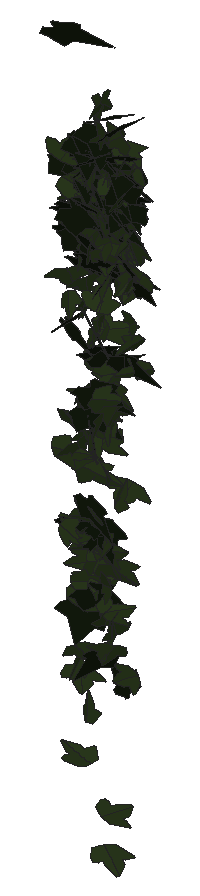
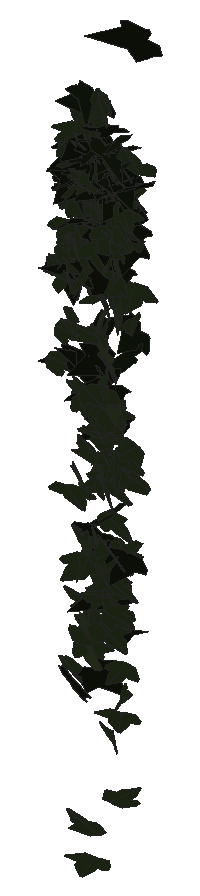
# SketchUp Ruby script. Lengths in millimetres.
U = 1.mm
M = Sketchup.active_model
def pt(a) = Geom::Point3d.new(a.map { |v| v * U })
def face(e, loops, mat)
  f = e.add_face(loops[0].map { |a| pt(a) })
  loops[1..].each { |l| e.add_face(l.map { |a| pt(a) }).erase! }
  f.material = f.back_material = mat if mat
  f
end
# faces: each face lists its corners as indices into pts; further lists are holes
def faces(e, pts, list, mat = nil) = list.each { |f| face(e, (f[0].is_a?(Array) ? f : [f]).map { |l| l.map { |i| pts[i] } }, mat) }
# xy, xz, yz: faces in a plane at the given z, y or x. An outline is a flat list of corners, or four numbers for a rectangle; further outlines are holes
def ring(l) = l.size == 4 ? [[l[0], l[1]], [l[2], l[1]], [l[2], l[3]], [l[0], l[3]]] : l.each_slice(2).to_a
def flat(e, list, mat, &to3) = list.each { |f| face(e, (f[0].is_a?(Array) ? f : [f]).map { |l| ring(l).map { |u, v| to3.(u, v) } }, mat) }
def xy(e, z, list, mat = nil) = flat(e, list, mat) { |x, y| [x, y, z] }
def xz(e, y, list, mat = nil) = flat(e, list, mat) { |x, z| [x, y, z] }
def yz(e, x, list, mat = nil) = flat(e, list, mat) { |y, z| [x, y, z] }
def lines(e, pts, list) = list.each { |a, b| e.add_line(pt(pts[a]), pt(pts[b])) }
# prism: a flat outline (further loops are holes) pulled along v
def prism(e, loops, v, mat = nil)
  f = face(e, loops, mat); d = Geom::Vector3d.new(v.map { |x| x * U })
  f.pushpull(f.normal.samedirection?(d) ? d.length : -d.length)
end
def box(e, o, s, mat = nil) = prism(e, [[o, [o[0] + s[0], o[1], o[2]], [o[0] + s[0], o[1] + s[1], o[2]], [o[0], o[1] + s[1], o[2]]]], [0, 0, s[2]], mat)
def at(x, y, z, deg = 0) = Geom::Transformation.translation(pt([x, y, z])) * Geom::Transformation.rotation(ORIGIN, Z_AXIS, deg.degrees)
def axes(o, x, y, z) = Geom::Transformation.new([*x, 0, *y, 0, *z, 0, *pt(o).to_a, 1])
def part(name) = M.definitions.add(name)
# library, detail: a bought-in or finely detailed component or shape, given as its bounding box
def library(name, o, s) = part(name).tap { |d| box(d.entities, o, s) }
def detail(e, o, s) = box(e.add_group.entities, o, s)
def put(e, d, t, mat = nil) = e.add_instance(d, t).tap { |i| i.material = mat if mat }
def group(e, t, mat = nil) = e.add_group.tap { |g| g.transformation = t; g.material = mat if mat }.entities
root = M.entities
M.materials.add("efeu1").color = [18, 25, 13]
M.materials.add("efeu2").color = [43, 57, 29]
c1 = part("ivyleaf_10")
p = [[0,12.8,-0.8],[-1.5,51.3,-10.9],[-4.9,51,-11.6],[-13.6,26.5,-7.3],[-13.2,15.9,-4.6],[-21.1,19.3,-7.2],
  [-29.5,16.3,-8.3],[-29.2,8.3,-6.2],[-19.7,-9.8,0.5],[-7.6,-13,4],[1,-12.2,5.8],[-0.4,51.1,-11.1],
  [-1.5,51.1,-10.9],[1,-12.4,5.9],[16.9,-12.4,3.5],[35.1,9.1,-5.1],[35,12.9,-6.1],[20.5,16.4,-4.9],
  [15.8,15,-3.8],[15.3,27.6,-7.1],[12.8,31.3,-7.8]]
faces(c1.entities,p,[[0,1,2,3,4,5,6,7,8,9,10],[11,12,0,13,14,15,16,17,18,19,20]],"efeu2")
c2 = part("ivyleaf_9")
p = [[39.1,54.8,31.7],[34.5,51.8,30.2],[-5.3,25.2,17.3],[-17.9,28.3,20.9],[-21.6,21.7,17],[-20.2,4.3,5.3],
  [-22.9,-0.3,2.5],[-17.1,-4,-0.6],[-2,-2.1,-1.2],[-0.7,-15.4,-10.1],[16.6,-22.3,-16.7],[21.1,-15.1,-12.5],
  [32.7,-10.7,-11],[46.1,-1.8,-6.6],[30.8,11.2,3.8]]
faces(c2.entities,p,[[0,1,2,3,4,5,6,7,8,9,10,11,12,13,14]],"efeu1")
put(root,c1,axes([2123.1,995.3,1030.1],[0.1906,0.68433,-0.17615],[-0.10749,-0.16959,-0.69095],[-1.34057,0.11089,0.03036]))
put(root,c1,axes([2125.7,988.9,1083.8],[-0.99593,-0.55975,-0.22734],[0.29957,0.16407,-0.76625],[1.11012,-0.54644,0.00281]))
put(root,c2,axes([2112.8,1000.5,1285.4],[0.02321,-0.74967,-0.23177],[0.08312,0.23208,-0.7484],[1.49109,-0.00127,0.04533]))
put(root,c1,axes([2135.8,1019.4,138.7],[0.62325,0.48649,0.41572],[-0.42495,-0.35077,0.58638],[1.14134,-0.39626,-0.00869]))
put(root,c1,axes([2116.7,1004.2,796.9],[-1.06583,0.27968,-0.34624],[0.60096,-0.14253,-0.62586],[-0.597,-0.6428,-0.01187]))
put(root,c1,axes([2133.1,1008.9,1242.5],[-0.27065,-0.75335,0.02688],[-0.01437,-0.02593,-0.76665],[1.43461,-0.14238,-0.00261]))
put(root,c1,axes([2133.3,1007.4,1229],[-0.52244,-0.70599,-0.01567],[0.01958,0.01282,-0.75747],[1.34384,-0.27465,0.00494]))
put(root,c1,axes([2102.9,999.1,731.2],[0.44156,-0.23226,-0.7183],[1.25411,-0.30437,0.31126],[-0.70107,-0.69076,0.10437]))
put(root,c2,axes([2126.7,1007.6,595.2],[1.22717,0.3981,-0.16174],[-0.27617,-0.07279,-0.75766],[-0.76976,0.66077,0.01398]))
put(root,c1,axes([2136.1,1008.7,1200.2],[-0.22378,-0.7354,0.18371],[-0.00371,-0.18561,-0.74427],[1.44263,-0.11455,0.02659]))
put(root,c2,axes([2113.8,1005.4,969.3],[0.92362,-0.62679,-0.07712],[-0.08881,0.0614,-0.79271],[1.19862,0.48754,0.00069]))
put(root,c1,axes([2125.4,1022,301.9],[1.17824,0.36942,0.04018],[0.0672,0.01923,-0.72092],[-0.70403,0.62009,-0.00157]))
put(root,c2,axes([2132.2,967.3,993.6],[0.46018,0.56096,0.59216],[0.42819,0.54781,-0.61081],[-1.49218,0.33019,0.00734]))
put(root,c1,axes([2142.9,1026.1,485.3],[-0.24172,-0.47422,0.54553],[-0.25536,-0.5288,-0.49091],[1.35179,-0.18469,0.00481]))
put(root,c1,axes([2121.2,985,1307.7],[1.44549,0.16265,-0.27372],[0.51115,0.05298,0.77672],[0.32546,-0.80558,-0.00418]))
put(root,c1,axes([2130.5,977.6,595.4],[-0.00655,0.62956,0.46716],[-0.00573,0.46715,-0.62957],[-1.49201,-0.00456,0.00037]))
put(root,c1,axes([2134.2,1010.4,326.8],[0.10382,0.30482,-0.67747],[-0.15658,-0.67264,-0.30927],[-1.40516,0.09747,-0.01559]))
put(root,c1,axes([2120.4,1016.4,708],[0.46974,-0.40499,-0.55279],[0.74794,-0.39768,0.46682],[-1.06843,-0.45645,0.08375]))
put(root,c1,axes([2141.8,994.7,756.5],[-0.48662,-0.77369,-0.37196],[0.19418,0.35797,-0.81472],[1.62223,-0.27493,-0.01405]))
put(root,c1,axes([2138.2,1015.5,847.5],[-0.26935,-0.35235,-0.59672],[-0.07607,-0.60387,0.36605],[-1.31668,0.10697,0.10092]))
put(root,c2,axes([2113.2,976.6,1550.7],[0.32292,0.23859,-0.77992],[0.84205,0.64229,0.29274],[1.30399,-0.47384,0.0041]))
put(root,c1,axes([2133.9,1002.4,588.8],[1.26574,0.16037,-0.13782],[0.25425,0.03394,0.68412],[0.31197,-0.67834,0.00164]))
put(root,c2,axes([2142.6,979.7,1166.2],[1.2367,0.10918,-0.4395],[-0.81863,-0.09161,-0.65872],[-0.26956,0.7791,-0.01587]))
put(root,c1,axes([2147.2,1006.1,1221.2],[-0.39847,-0.74045,0.0741],[-0.00265,-0.07659,-0.76923],[1.41625,-0.20847,0.01941]))
put(root,c2,axes([2157.8,999.7,1299.3],[0.47799,0.63308,-0.36755],[-0.67575,-0.23447,-0.64646],[-1.21837,0.37841,0.21435]))
put(root,c1,axes([2141.7,1033,569.8],[-0.05482,-0.12579,0.72322],[0.29785,-0.70819,-0.11695],[1.36497,0.14948,0.05457]))
put(root,c2,axes([2159.1,1006.5,1157.3],[-0.04924,0.08797,-0.81043],[-1.29872,0.44124,0.06968],[0.84874,0.68027,0.05961]))
put(root,c1,axes([2143,1015.2,1107.8],[-1.21258,0.36168,-0.0914],[0.13738,-0.05795,-0.73248],[-0.69658,-0.64103,0.01465]))
put(root,c2,axes([2118.9,984.6,1205.7],[1.17553,0.0895,0.47053],[0.86138,0.14223,-0.62117],[-0.29832,0.76333,0.06057]))
put(root,c2,axes([2162.2,992.1,1298.4],[-0.68201,0.68144,0.00431],[-0.00369,0.00385,-0.76992],[-1.29694,-0.35835,-0.00007]))
put(root,c1,axes([2166,1016.1,446.2],[-1.00082,-0.28656,0.45055],[-0.75452,-0.21406,-0.59887],[0.68074,-0.65856,-0.00139]))
put(root,c1,axes([2155.7,1021.7,837.1],[-0.36986,-0.36266,-0.60894],[-0.56519,-0.53165,0.4114],[-1.22477,0.35485,-0.00596]))
put(root,c2,axes([2145.3,993.3,1262.7],[0.74221,0.68815,0.26433],[0.24238,0.23165,-0.79097],[-1.38189,0.41023,0.00323]))
put(root,c2,axes([2148,991.1,1266.2],[-0.42561,0.72543,-0.3368],[-0.37212,0.28952,0.75342],[1.476,0.28217,0.09283]))
put(root,c1,axes([2152.7,1022.4,956.7],[0.42982,-0.64894,-0.08842],[-0.07411,0.08006,-0.68703],[1.24426,0.22894,-0.01038]))
put(root,c1,axes([2167.9,1006.7,536],[1.01125,-0.02957,-0.57194],[-1.08021,0.07698,-0.53127],[0.14553,0.77686,0.03087]))
put(root,c1,axes([2152,1015,773.9],[-0.55001,-0.67888,-0.2729],[0.19736,0.25245,-0.73782],[1.37847,-0.30702,-0.00325]))
put(root,c1,axes([2127.2,994.5,1184.1],[0.96208,-0.07101,0.60035],[1.14358,-0.02705,-0.50914],[0.12653,0.78437,0.0368]))
put(root,c1,axes([2164.3,1013.3,851.3],[-1.03656,-0.5294,0.27577],[-0.34253,-0.2103,-0.75917],[1.0832,-0.57311,0.02383]))
put(root,c1,axes([2147.3,989.4,369.2],[-0.72212,-0.41519,-0.37968],[0.49988,0.27427,-0.5624],[0.94693,-0.4614,0.00735]))
put(root,c1,axes([2156.6,1013.2,1192.5],[-1.15405,-0.43398,0.13134],[0.06766,-0.26416,-0.70869],[0.8603,-0.56139,0.23193]))
put(root,c2,axes([2177.1,998.4,590],[-0.88251,0.24143,-0.6951],[-1.21878,0.27227,0.52177],[0.68978,0.78996,0.0326]))
put(root,c2,axes([2150.6,1002.2,435],[-0.65061,-0.74582,0.11068],[-0.08528,-0.10121,-0.82043],[1.43245,-0.34477,0.00143]))
put(root,c1,axes([2157.8,1004.9,234.4],[0.95533,-0.45893,0.37581],[-0.52998,0.25238,0.68013],[-0.99679,-0.57402,-0.00143]))
put(root,c1,axes([2150.6,1007.2,1266.6],[-1.36192,-0.17808,-0.21029],[0.40464,0.01545,-0.73659],[0.33363,-0.74569,0.03496]))
put(root,c1,axes([2157.8,998.6,1173.6],[0.95469,-0.56592,-0.14151],[-0.11647,0.13455,-0.75503],[1.10409,0.50353,0.04271]))
put(root,c1,axes([2175.1,1006.7,574.7],[-0.55584,-0.33727,0.57779],[-0.73016,-0.43207,-0.44612],[1.04314,-0.48214,-0.00439]))
put(root,c1,axes([2163.7,1028.7,589.6],[-0.03045,0.00559,-0.7466],[-0.55334,-0.68787,0.00108],[-1.30881,0.29069,0.01691]))
put(root,c1,axes([2150.5,1000.7,1136.1],[0.27502,-0.54934,0.56919],[0.50438,-0.51155,-0.56099],[1.41851,0.2884,0.08912]))
put(root,c1,axes([2161.7,988.1,1045.2],[0.11245,-0.70184,-0.30774],[-0.03305,0.30735,-0.70428],[1.45814,0.06109,0.00777]))
put(root,c1,axes([2179.7,984.4,635.4],[-0.77726,0.02461,0.55664],[-1.059,0.01796,-0.40903],[-0.05528,-0.69016,0.00921]))
put(root,c2,axes([2150.1,1004.3,1279.9],[-0.3023,-0.75624,0.07728],[0.00329,-0.07931,-0.77254],[1.44677,-0.15784,0.0179]))
put(root,c2,axes([2151.9,1009.2,1305.1],[-0.35871,-0.55904,0.48848],[0.02664,-0.50656,-0.57433],[1.41265,-0.1324,0.13487]))
put(root,c1,axes([2148.3,988.7,1244.1],[-1.05643,0.30851,-0.44186],[0.6171,-0.31547,-0.62759],[-0.81921,-0.63548,0.09704]))
put(root,c1,axes([2164.8,983.9,1293],[1.01221,-0.50481,-0.2839],[-0.26448,0.26295,-0.72789],[1.07006,0.54251,0.08864]))
put(root,c2,axes([2175.6,997.9,1336.1],[-0.1106,0.75019,0.17904],[-0.21673,0.16924,-0.74607],[-1.45178,-0.08242,0.09774]))
put(root,c1,axes([2163,990.3,1034.1],[0.30569,-0.689,-0.23034],[0.01283,0.2373,-0.70514],[1.38258,0.15014,0.05747]))
put(root,c1,axes([2141.8,975.3,1266.6],[0.67684,0.39365,0.6463],[0.6837,0.54069,-0.52701],[-1.26761,0.50182,0.06084]))
put(root,c1,axes([2164.2,988.7,1082.4],[-0.54356,-0.66197,-0.21211],[0.14198,0.1988,-0.72089],[1.31532,-0.29502,-0.00984]))
put(root,c2,axes([2147.3,1005.5,1267],[0.48446,-0.68257,-0.23231],[0.0207,0.24997,-0.72254],[1.37209,0.23723,0.09293]))
put(root,c2,axes([2145.1,1005.3,1168.3],[0.49786,-0.68256,0.21834],[0.18302,-0.19689,-0.73074],[1.35156,0.27809,0.01853]))
put(root,c1,axes([2147.6,1032.1,914.7],[0.26893,-0.3027,0.65661],[0.96544,-0.43522,-0.30981],[0.98053,0.51155,0.12495]))
put(root,c1,axes([2166.1,1020.1,969.5],[0.49961,-0.6428,0.0458],[0.00844,-0.04765,-0.6942],[1.22645,0.26218,-0.01388]))
put(root,c1,axes([2169.2,1014.8,718.8],[0.54966,-0.68795,-0.15673],[-0.13164,0.14093,-0.74606],[1.3364,0.29684,-0.00903]))
put(root,c1,axes([2162.1,1004,1246.7],[0.99154,0.5584,-0.11091],[-0.16275,-0.07188,-0.76358],[-1.07121,0.52779,0.01335]))
put(root,c2,axes([2158.4,994.6,1333],[-0.33593,-0.75548,0.0174],[-0.00848,-0.01683,-0.77582],[1.43818,-0.17656,-0.00051]))
put(root,c1,axes([2172.8,987.7,1287.6],[0.72146,-0.62975,-0.27747],[-0.28767,0.23285,-0.73499],[1.27773,0.408,-0.00881]))
put(root,c1,axes([2187.9,1004.8,1153],[-0.5211,-0.07845,0.70308],[-0.92598,-0.52641,-0.24821],[0.97742,-0.54053,0.13969]))
put(root,c2,axes([2140.2,986.9,1218.1],[1.39496,-0.16802,0.24714],[0.45701,-0.05855,-0.75196],[0.33857,0.77128,-0.00324]))
put(root,c2,axes([2152,987.6,1166.4],[-0.07833,-0.51639,-0.61805],[0.27497,0.60408,-0.51434],[1.50793,-0.13698,0.06168]))
put(root,c1,axes([2169.5,999.3,1291.4],[-0.74225,-0.67294,-0.075],[0.16784,0.03533,-0.77559],[1.27768,-0.39557,0.05832]))
put(root,c1,axes([2176.8,1000.4,1243.2],[-1.14097,-0.44929,0.13192],[-0.19486,-0.08335,-0.74915],[0.86962,-0.60816,0.00522]))
put(root,c1,axes([2176.6,1019.9,1154.6],[-1.1965,-0.35651,0.14177],[-0.18423,-0.11595,-0.72085],[0.70657,-0.63395,0.05212]))
put(root,c1,axes([2156.4,1008.8,1308.5],[0.48105,-0.34799,0.63465],[0.71639,-0.51097,-0.43009],[1.17658,0.4534,0.0024]))
put(root,c1,axes([2169.5,1006.3,1270.5],[0.75682,-0.64727,-0.14511],[0.02721,0.17751,-0.75262],[1.26217,0.38429,0.10323]))
put(root,c1,axes([2183.6,1010.9,787.2],[1.0368,-0.07923,0.49181],[-0.92923,0.05969,0.55044],[-0.18813,-0.7315,-0.00835]))
put(root,c1,axes([2157.1,984.8,462.7],[1.25407,0.02388,-0.25657],[0.48791,0.01044,0.65936],[0.04956,-0.70704,0.00107]))
put(root,c2,axes([2154.3,1012.9,787.8],[0.02629,0.00313,-0.8044],[1.3086,-0.41761,0.01018],[-0.79459,-0.68765,-0.00985]))
put(root,c2,axes([2151.6,971.5,1220],[0.56113,-0.24248,-0.87086],[-0.02541,0.91474,-0.25922],[1.72029,0.0926,0.28023]))
put(root,c1,axes([2147.5,1012.8,816.4],[0.21865,-0.02257,0.68917],[1.06707,0.40976,-0.08004],[-0.76393,0.56591,0.08545]))
put(root,c1,axes([2183.9,988.4,1180.5],[-0.95323,-0.48174,0.2918],[-0.38061,-0.21293,-0.6948],[1.00207,-0.53913,0.01368]))
put(root,c2,axes([2159.7,1007.2,1259.6],[0.04829,-0.77043,-0.00224],[0.0002,0.00225,-0.77085],[1.46629,0.02537,0.00018]))
put(root,c1,axes([2158,979,503.9],[-0.09041,-0.0901,0.69977],[0.55632,0.63582,0.10171],[-1.22213,0.29609,-0.00547]))
put(root,c2,axes([2153.6,993.2,1348.2],[0.69333,-0.67624,-0.17594],[0.03274,0.20703,-0.76013],[1.32945,0.34757,0.11047]))
put(root,c1,axes([2164.2,1001.1,537.2],[-0.03287,-0.28581,-0.75932],[0.64334,0.6879,-0.26662],[1.40372,-0.32196,0.10441]))
put(root,c1,axes([2192.6,1003.3,714.8],[-0.39342,0.40739,-0.74788],[-0.74515,0.63798,0.45575],[1.4394,0.44162,0.03152]))
put(root,c1,axes([2171.8,1019,1161.8],[-1.28943,0.21779,0.21168],[0.35295,-0.11315,0.70997],[0.45776,0.70073,0.04885]))
put(root,c1,axes([2174.1,984.7,1151],[0.41329,-0.55667,-0.48039],[0.12294,0.51341,-0.56573],[1.39401,0.11976,0.19232]))
put(root,c1,axes([2170.1,1004.1,769.4],[0.096,0.73022,-0.15348],[-0.03878,-0.15243,-0.73189],[-1.41959,0.05355,0.00962]))
put(root,c1,axes([2191,994.7,1289.3],[0.73216,-0.29258,-0.59439],[-0.7721,0.43936,-0.47883],[0.99681,0.55521,0.06569]))
put(root,c1,axes([2181.4,1003.6,1157.1],[0.66119,-0.52139,-0.44504],[-0.19088,0.4549,-0.61123],[1.29059,0.3344,0.13759]))
put(root,c1,axes([2177.9,1004.1,1266.5],[0.49628,-0.72266,0.08953],[0.04653,-0.08636,-0.76825],[1.38511,0.26183,-0.00627]))
put(root,c1,axes([2173.1,994.7,1264.8],[-0.46184,0.69755,-0.19782],[0.05112,-0.19981,-0.73753],[-1.37898,-0.24103,0.03891]))
put(root,c1,axes([2178.7,983.8,1228.1],[-1.18814,0.42429,0.02489],[-0.04017,0.01322,-0.75482],[-0.8079,-0.62464,0.00093]))
put(root,c2,axes([2185.6,1000.6,1179.9],[0.94848,0.36695,-0.44053],[-0.83376,-0.13283,-0.60623],[-0.70393,0.65176,0.12447]))
put(root,c1,axes([2183.1,1007,1222.1],[-0.92806,-0.57572,0.15636],[0.03729,-0.2173,-0.73897],[1.13479,-0.46369,0.15216]))
put(root,c2,axes([2187.1,1010.8,362.1],[-0.17551,0.37815,-0.77973],[0.32176,-0.76122,-0.38917],[-1.61761,-0.19245,0.00719]))
put(root,c2,axes([2162.3,999.3,1275.4],[1.46887,0.05925,-0.00001],[-0.01481,0.10124,-0.76737],[-0.11179,0.76512,0.10154]))
put(root,c2,axes([2156.2,1007.1,1267.3],[0.97918,-0.57132,0.06293],[0.1617,-0.00793,-0.76667],[1.0819,0.51827,0.05764]))
put(root,c2,axes([2167.2,992.9,830.1],[0.0486,-0.42179,-0.76247],[-0.05173,0.76204,-0.42246],[1.65756,0.03615,0.00917]))
put(root,c2,axes([2185.3,986.3,1330.6],[0.75333,0.6132,-0.26896],[-0.31625,-0.21271,-0.7295],[-1.23451,0.42869,0.02275]))
put(root,c1,axes([2158.6,1001.8,589.5],[0.89619,0.11639,0.50683],[0.9124,0.16773,-0.48393],[-0.38344,0.67117,0.03305]))
put(root,c1,axes([2184.7,1008.9,990.1],[0.79388,-0.58263,-0.14501],[-0.16636,0.11576,-0.71655],[1.13052,0.42618,-0.00361]))
put(root,c2,axes([2156,986.3,1118.6],[1.48777,0.09078,0.29446],[0.55767,0.02943,-0.78696],[-0.18145,0.83482,-0.00428]))
put(root,c1,axes([2175.5,999.6,915.4],[1.33026,-0.30376,-0.00274],[0.0157,0.01211,0.76198],[-0.57792,-0.69886,0.01439]))
put(root,c1,axes([2185.7,997.7,1057.3],[0.64577,-0.66324,-0.11644],[-0.08367,0.10828,-0.74493],[1.27885,0.342,0.01006]))
put(root,c1,axes([2184.6,997.6,1014.8],[0.28272,-0.25111,-0.68556],[0.0687,0.70127,-0.24904],[1.38782,0.01644,0.15199]))
put(root,c2,axes([2183.4,971.1,1323.4],[0.53165,0.64425,0.33928],[0.23426,0.31637,-0.70211],[-1.36582,0.30504,0.01164]))
put(root,c2,axes([2166.4,992.6,651.7],[0.55686,-0.81264,-0.10232],[-0.071,0.09532,-0.8637],[1.55721,0.29495,-0.00279]))
put(root,c2,axes([2168.1,998.6,939.1],[0.96516,0.41395,0.46497],[0.70093,0.28402,-0.65454],[-0.95523,0.62666,-0.01049]))
put(root,c1,axes([2187.3,1029.1,888.7],[-0.44785,-0.55966,0.43975],[0.08175,-0.47348,-0.57961],[1.35216,-0.15674,0.18069]))
put(root,c1,axes([2186.7,997,1421.5],[0.70796,-0.66538,-0.21572],[-0.0477,0.23149,-0.75724],[1.33038,0.36238,0.08764]))
put(root,c1,axes([2175.3,1002.8,985.1],[0.11279,-0.18184,0.72332],[0.68897,-0.62738,-0.18738],[1.24104,0.36482,0.03829]))
put(root,c1,axes([2169.9,995.4,715.2],[-0.7575,-0.32731,-0.64646],[1.05864,0.33466,-0.51191],[0.88379,-0.68141,0.0591]))
put(root,c1,axes([2178.3,1007.7,583.9],[0.69578,-0.67525,-0.10081],[0.10554,-0.08461,0.76781],[-1.29508,-0.36967,0.00841]))
put(root,c1,axes([2188.6,998.3,1424.9],[-0.2161,-0.54971,-0.65849],[0.2113,0.64923,-0.56112],[1.6188,-0.15813,-0.01466]))
put(root,c1,axes([2181.8,1005.5,1252],[-1.10225,-0.4464,-0.25896],[0.6301,-0.02278,-0.70116],[0.75344,-0.63401,0.20752]))
put(root,c1,axes([2186.6,998.5,872.7],[-1.01391,-0.54992,-0.3576],[0.44192,0.27276,-0.76536],[1.16759,-0.58077,-0.02085]))
put(root,c1,axes([2193.3,1008.2,1245.4],[0.51263,-0.70136,-0.16635],[0.00118,0.17781,-0.74867],[1.37185,0.26193,0.0628]))
put(root,c1,axes([2196.1,1004.6,1280],[-0.68969,-0.6775,-0.10906],[0.09125,0.09803,-0.76832],[1.30283,-0.36552,-0.00392]))
put(root,c2,axes([2205.4,982.4,970.4],[0.0937,-0.60373,0.60557],[-0.12543,0.60209,0.60562],[-1.62259,-0.08141,-0.01185]))
put(root,c2,axes([2176.9,982.1,490.8],[0.0779,-0.11735,-0.80752],[0.17858,0.80385,-0.11206],[1.54272,-0.08713,0.05375]))
put(root,c1,axes([2208.2,992.6,1245.3],[-1.22569,0.18696,0.35491],[-0.68889,0.0185,-0.66657],[-0.32907,-0.7351,0.07349]))
put(root,c1,axes([2197.5,981.9,1390.3],[-0.94538,0.63448,0.0429],[-0.26187,-0.05409,-0.79328],[-1.18163,-0.49564,0.14148]))
put(root,c2,axes([2182.8,1003.4,613.1],[-0.96925,-0.22396,-0.63282],[1.11981,0.23345,-0.55613],[0.61501,-0.77802,0.01529]))
put(root,c1,axes([2185.5,992.9,492.9],[0.30836,0.2122,-0.76491],[0.62743,0.69219,0.26186],[1.37432,-0.36362,0.05208]))
put(root,c1,axes([2194.5,992.7,825.4],[0.255,-0.61287,0.3068],[0.19214,-0.29155,-0.62649],[1.29017,0.16455,0.03266]))
put(root,c2,axes([2193.4,998.2,1365.5],[-0.71121,-0.68913,-0.10923],[0.12241,0.08936,-0.78381],[1.32227,-0.37893,0.01381]))
put(root,c1,axes([2181.5,1018.5,761.6],[1.20984,-0.18503,-0.31988],[0.58245,-0.09313,0.66206],[-0.39418,-0.70551,-0.00351]))
put(root,c2,axes([2197.6,981.8,1076.3],[0.22269,0.22287,0.77167],[0.49419,0.72745,-0.24947],[-1.44659,0.28282,0.03357]))
put(root,c2,axes([2215.9,997.6,1214.4],[-0.56237,0.69132,0.10974],[-0.13024,0.09002,-0.75133],[-1.32581,-0.30208,0.02725]))
put(root,c1,axes([2203,1012.9,1141.1],[-1.04802,-0.49841,-0.0058],[0.00758,0.00425,-0.74272],[0.9486,-0.55068,-0.00048]))
put(root,c1,axes([2210.9,980.2,1173.2],[0.77695,-0.5559,-0.49614],[-0.57296,0.39444,-0.68965],[1.29718,0.50718,-0.00745]))
put(root,c1,axes([2188.2,1007.3,371.7],[0.35561,-0.71932,-0.25458],[0.27149,-0.22455,0.73917],[-1.42661,-0.22204,0.07721]))
put(root,c1,axes([2195.9,985.9,1045.1],[0.72784,0.66246,-0.36227],[0.29112,0.3297,0.76436],[1.40721,-0.41085,0.02925]))
put(root,c1,axes([2196.6,1007.3,1087.2],[0.02764,-0.60516,0.47972],[0.38609,-0.45996,-0.58638],[1.4181,0.13702,0.1503]))
put(root,c2,axes([2183.5,981.3,881.2],[0.08152,-0.2263,-0.77949],[0.31925,0.76619,-0.21322],[1.51144,-0.14963,0.08708]))
put(root,c1,axes([2190.6,999.3,1140.7],[1.37923,-0.04449,0.22869],[0.43373,-0.01976,-0.72603],[0.09205,0.75966,-0.0055]))
put(root,c1,axes([2201.6,1011.5,1220.9],[1.01797,-0.54169,-0.03414],[0.11055,0.10479,-0.75255],[1.02706,0.52562,0.11484]))
put(root,c1,axes([2202.4,1007,1299.1],[-1.07284,0.51328,-0.09591],[0.10259,-0.08318,-0.76197],[-0.98848,-0.56572,0.02501]))
put(root,c1,axes([2217.7,976.6,516.9],[0.463,-0.34808,-0.70701],[-0.51609,0.65777,-0.41714],[1.40823,0.3555,0.07958]))
put(root,c1,axes([2202.3,994.9,1309.3],[0.83177,-0.62924,0.18954],[0.20763,-0.155,-0.76612],[1.23336,0.45045,0.00115]))
put(root,c1,axes([2203.7,996.8,435.1],[-0.54556,-0.63728,-0.08889],[-0.02211,-0.09217,0.69826],[-1.22441,0.28561,0.027]))
put(root,c1,axes([2215.7,995.2,388.4],[-0.87986,-0.54099,0.17519],[-0.20398,-0.13885,-0.71156],[1.06285,-0.47449,0.00847]))
put(root,c1,axes([2195,1009.2,815.5],[0.86133,-0.45606,0.49666],[0.66542,-0.35274,-0.6425],[1.0973,0.57189,-0.00023]))
put(root,c1,axes([2213,997.7,1371.8],[-0.56541,-0.72355,-0.03236],[0.00584,0.03372,-0.7821],[1.37843,-0.29693,-0.00996]))
put(root,c2,axes([2176.9,1014.9,1105.1],[0.40855,0.06139,-0.8254],[1.07966,0.61001,0.19291],[1.14705,-0.59604,0.11241]))
put(root,c2,axes([2212.5,979.6,1409.4],[0.68089,0.63808,0.28206],[-0.07228,0.33433,-0.70815],[-1.32578,0.30948,0.18346]))
put(root,c1,axes([2207.5,998.9,1294],[-1.11273,0.51066,-0.08668],[0.13231,-0.05216,-0.77625],[-0.97686,-0.58874,-0.0064]))
put(root,c1,axes([2211.4,977.5,1215.5],[-0.24553,0.63164,0.40942],[-0.2557,0.38939,-0.64309],[-1.40958,-0.18066,0.04534]))
put(root,c2,axes([2191.8,998.8,919],[0.03699,-0.0347,0.76344],[1.375,0.24983,-0.00704],[-0.47422,0.72167,0.03915]))
put(root,c1,axes([2186,1011.9,985.5],[0.70331,-0.09053,-0.64841],[1.23932,0.12791,0.35326],[0.129,-0.73528,0.14129]))
put(root,c1,axes([2213,1010.9,411.7],[-0.39562,-0.64513,-0.35991],[-0.23494,-0.33829,0.67768],[-1.38618,0.24146,-0.01214]))
put(root,c1,axes([2219.6,997.7,847.1],[-0.73337,-0.60102,0.0939],[-0.0927,-0.08031,-0.71394],[1.15402,-0.3884,0.00232]))
put(root,c1,axes([2207.1,1010.1,430.6],[0.06475,-0.40387,-0.6787],[0.09063,-0.67704,0.40527],[-1.50036,-0.05832,-0.00481]))
put(root,c1,axes([2212.1,1018,1080.3],[-0.10512,0.71756,-0.02859],[-0.11244,-0.03311,-0.71706],[-1.3621,-0.05264,0.0614]))
put(root,c1,axes([2219,1000.9,548.5],[-0.24853,0.40394,0.56917],[-0.43256,0.52288,-0.42323],[-1.25593,-0.26002,0.03313]))
put(root,c1,axes([2211.5,1003,589.4],[0.13763,-0.35282,0.70235],[0.32744,-0.6811,-0.35986],[1.4596,0.18606,0.01451]))
put(root,c1,axes([2222.2,1007.7,1217.4],[-0.81626,-0.59636,0.21067],[-0.11533,-0.21463,-0.73091],[1.19819,-0.42692,0.07317]))
put(root,c1,axes([2218.5,1001.2,1254.8],[-0.06262,-0.6402,0.41441],[0.05549,-0.41555,-0.63964],[1.45036,-0.01174,0.04237]))
put(root,c1,axes([2203.1,997.6,-6.8],[1.08284,0.46628,0.22921],[0.33399,0.14748,-0.73561],[-0.93074,0.5954,0.0027]))
put(root,c2,axes([2197.6,997.5,1247.8],[0.5633,-0.69904,-0.00213],[0.07231,0.0184,-0.75794],[1.32845,0.29541,0.04216]))
put(root,c1,axes([2198.8,999.1,1255.5],[1.065,0.2124,-0.49753],[0.83585,0.2396,0.59624],[0.60117,-0.70941,0.05241]))
put(root,c1,axes([2195.9,1009.4,57.2],[0.98497,-0.03304,-0.47466],[0.90417,-0.00288,0.51819],[-0.05005,-0.70223,0.02021]))
put(root,c1,axes([2203.6,972.4,874.5],[-0.2548,-0.21487,-0.80094],[0.89747,0.64764,-0.25257],[1.29824,-0.48988,0.0174]))
put(root,c1,axes([2237.5,987.1,1378.1],[-0.91719,0.36232,0.49663],[-1.03667,0.04088,-0.55839],[-0.5424,-0.69081,0.22743]))
put(root,c2,axes([2216.4,1002.6,1280],[-0.88101,-0.60795,-0.10425],[0.14022,0.07492,-0.76401],[1.16553,-0.46855,0.01311]))
put(root,c2,axes([2199.2,1010.1,1199.8],[0.33384,-0.56337,-0.47937],[0.28181,0.50944,-0.54452],[1.37933,0.03227,0.22727]))
put(root,c2,axes([2202,1003.9,1323.9],[0.98661,-0.54014,-0.2023],[-0.17277,0.19221,-0.7458],[1.08404,0.52222,0.06526]))
put(root,c1,axes([2207.1,984.1,1153.5],[-0.7548,-0.30421,-0.61536],[0.96118,0.35203,-0.49952],[0.88485,-0.6419,0.01769]))
put(root,c1,axes([2196.8,997.1,571.8],[0.61027,-0.23828,-0.71476],[1.04555,-0.45766,0.39903],[-0.98131,-0.6358,-0.01935]))
put(root,c1,axes([2223.7,1015.6,1172.8],[-0.81024,-0.60612,-0.08955],[0.2228,0.02657,-0.73637],[1.14461,-0.43423,0.07995]))
put(root,c2,axes([2243.2,1005.4,315.9],[-0.1205,0.2723,0.7111],[-0.46066,0.66935,-0.27786],[-1.37403,-0.24829,0.0308]))
put(root,c1,axes([2238.6,1006.3,1153.1],[-0.13127,0.39523,0.63222],[-0.89794,0.4685,-0.34435],[-1.09877,-0.43008,0.20588]))
put(root,c1,axes([2228.2,1024.4,690.9],[1.39379,0.08478,-0.17386],[-0.33076,-0.01055,-0.73718],[-0.16165,0.75262,0.00925]))
put(root,c1,axes([2218.9,997.5,545.2],[-1.08504,-0.40213,-0.4742],[0.72376,0.28346,-0.69759],[0.93616,-0.68523,-0.01029]))
put(root,c1,axes([2208.9,1012.9,871.9],[-0.25907,0.09116,-0.71728],[0.83749,-0.5687,-0.15579],[-1.09192,-0.45782,0.0507]))
put(root,c2,axes([2218,982.8,1330.9],[0.96072,0.51406,0.27066],[0.39472,0.17547,-0.72008],[-1.03282,0.54524,-0.02344]))
put(root,c1,axes([2219.9,993.7,1284],[0.97747,0.65355,0.1581],[0.20053,0.11827,-0.83115],[-1.26391,0.5242,-0.0096]))
put(root,c2,axes([2204.3,1016.5,934],[0.0382,0.03924,-0.75868],[1.17951,0.43809,0.03906],[0.8362,-0.61974,-0.02043]))
put(root,c1,axes([2238.4,994.5,1215.8],[-1.05949,-0.4853,0.09085],[-0.12241,-0.06447,-0.7385],[0.93166,-0.56036,0.00629]))
put(root,c1,axes([2239.4,1016.1,1011.9],[0.62266,-0.42733,-0.45695],[-0.3614,0.42351,-0.53201],[1.13453,0.36943,0.08132]))
put(root,c1,axes([2234.2,1023.7,1086],[0.63892,-0.63345,-0.05716],[-0.01546,0.06036,-0.71661],[1.21039,0.33515,0.02102]))
put(root,c2,axes([2226.4,972.1,1389],[-0.17704,0.65707,-0.46318],[-0.19001,0.45322,0.66299],[1.51817,0.13335,0.02897]))
put(root,c1,axes([2240,1021.8,1137.5],[-0.58406,-0.6016,0.29864],[-0.05664,-0.31583,-0.66682],[1.27702,-0.28916,0.10701]))
put(root,c1,axes([2212.6,987.6,461.7],[0.80722,-0.03663,-0.54328],[1.03631,0.02951,0.42311],[0.00147,-0.6886,0.04703]))
put(root,c2,axes([2225.1,996.8,1259.2],[1.19842,0.41873,0.08048],[0.15228,0.02495,-0.75584],[-0.79711,0.63432,-0.0234]))
put(root,c1,axes([2233.4,1014.1,1158.6],[0.11605,0.73613,0.11685],[-0.09636,0.12106,-0.73623],[-1.41526,0.05212,0.05971]))
put(root,c1,axes([2236.7,996.8,1335.2],[0.54408,-0.73114,0.05065],[0.09157,-0.03552,-0.7844],[1.39184,0.28815,0.03181]))
put(root,c2,axes([2239.8,1006.4,1245.1],[-1.0532,-0.53924,-0.0067],[0.04411,-0.01419,-0.77222],[1.02542,-0.55324,0.02634]))
put(root,c2,axes([2231.8,992.8,1145.2],[1.17271,-0.18002,-0.4099],[-0.74846,0.11558,-0.64194],[0.40716,0.73098,0.00055]))
put(root,c1,axes([2253.8,1021.2,1102.6],[-1.15812,0.24593,0.34474],[-0.7746,-0.17298,-0.59501],[-0.22258,-0.67765,0.277]))
put(root,c1,axes([2234.4,1017.9,1168.4],[0.11225,-0.24793,0.70378],[0.31017,-0.68465,-0.25484],[1.38582,0.17332,0.00004]))
put(root,c2,axes([2251.5,977.5,1274.1],[-1.37674,0.34776,-0.12421],[-0.22102,0.04509,0.80258],[0.66714,0.73258,0.00956]))
put(root,c1,axes([2234.4,1011.4,1244.7],[-0.21852,0.73255,0.17535],[-0.03033,0.17498,-0.74141],[-1.43326,-0.11539,-0.01105]))
put(root,c2,axes([2246.7,1008.9,1096],[1.00106,0.1335,-0.60109],[-1.12729,-0.10625,-0.54191],[-0.32013,0.79163,0.02864]))
put(root,c1,axes([2242.8,1011.5,1099.7],[0.44882,0.47254,-0.49065],[-0.50177,-0.41545,-0.52682],[-1.19542,0.35179,0.03691]))
put(root,c1,axes([2242.3,987.9,1266.6],[0.08707,-0.7902,-0.24837],[0.02632,0.24944,-0.79106],[1.57622,0.03949,0.02693]))
put(root,c1,axes([2242.2,1028,1079],[-0.46877,-0.41245,0.52778],[0.09756,-0.57229,-0.42331],[1.27108,-0.10818,0.22714]))
put(root,c1,axes([2226.7,1019.5,1105.4],[-1.11561,0.09175,-0.43939],[0.7998,-0.14177,-0.59024],[-0.30019,-0.71872,0.06034]))
put(root,c2,axes([2222.4,998,1305.3],[1.42477,-0.18729,-0.03452],[-0.06304,0.00981,-0.77169],[0.35692,0.74935,0.00147]))
put(root,c1,axes([2252.7,999.4,346.4],[0.88119,-0.39093,-0.41607],[-0.62977,0.25279,-0.60574],[0.88544,0.56885,-0.01676]))
put(root,c1,axes([2242.2,1012.2,1095.5],[0.24509,-0.69831,-0.12199],[0.12311,0.13505,-0.70476],[1.34352,0.11501,0.08683]))
put(root,c1,axes([2255.9,1030,923.4],[-0.21147,-0.26039,0.66905],[-0.53847,-0.60634,-0.28297],[1.2558,-0.30384,-0.00867]))
put(root,c2,axes([2240.8,999.7,1322.6],[-0.77722,-0.67211,-0.04345],[0.03294,0.04032,-0.78643],[1.28141,-0.4087,-0.00614]))
put(root,c1,axes([2236.9,985.8,680.3],[0.85606,-0.67197,0.0682],[-0.05329,0.06332,0.80854],[-1.28437,-0.45052,0.01191]))
put(root,c1,axes([2249.3,1018.7,980.4],[-0.10778,-0.4593,0.55048],[-0.16232,-0.54395,-0.46263],[1.35477,-0.10171,-0.01164]))
put(root,c2,axes([2253.6,1000.4,1249.5],[-1.43519,-0.12576,-0.12036],[0.22062,0.03639,-0.76433],[0.24714,-0.76277,-0.01662]))
put(root,c2,axes([2233.8,1006.8,1258.2],[0.0876,-0.75714,-0.1445],[-0.02141,0.14409,-0.75853],[1.46684,0.04732,-0.00244]))
put(root,c1,axes([2250.4,997.4,1312.1],[-0.63596,-0.69594,-0.06383],[0.03834,0.06113,-0.77196],[1.32951,-0.33466,-0.00827]))
put(root,c1,axes([2248.3,1010,1168.1],[-1.26807,0.32126,0.02524],[-0.045,0.00907,-0.73969],[-0.61165,-0.6667,0.0021]))
put(root,c1,axes([2247.4,1000.3,1318.4],[1.38722,-0.26896,-0.11241],[-0.21029,0.02521,-0.77679],[0.5134,0.73707,-0.01445]))
put(root,c1,axes([2237.9,998.9,1352.6],[0.53914,0.64872,0.34617],[0.18994,0.33362,-0.70686],[-1.38648,0.29796,0.03777]))
